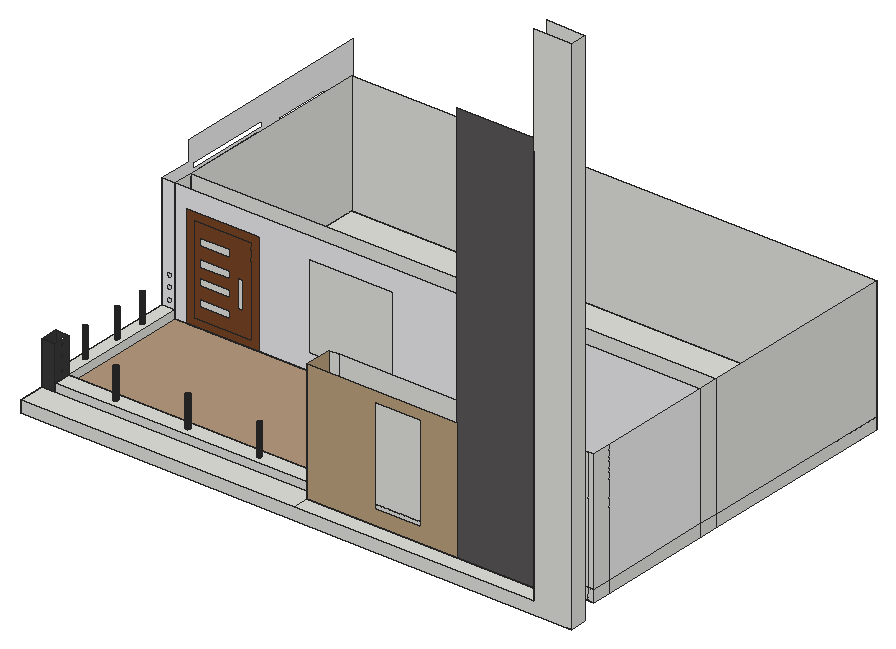
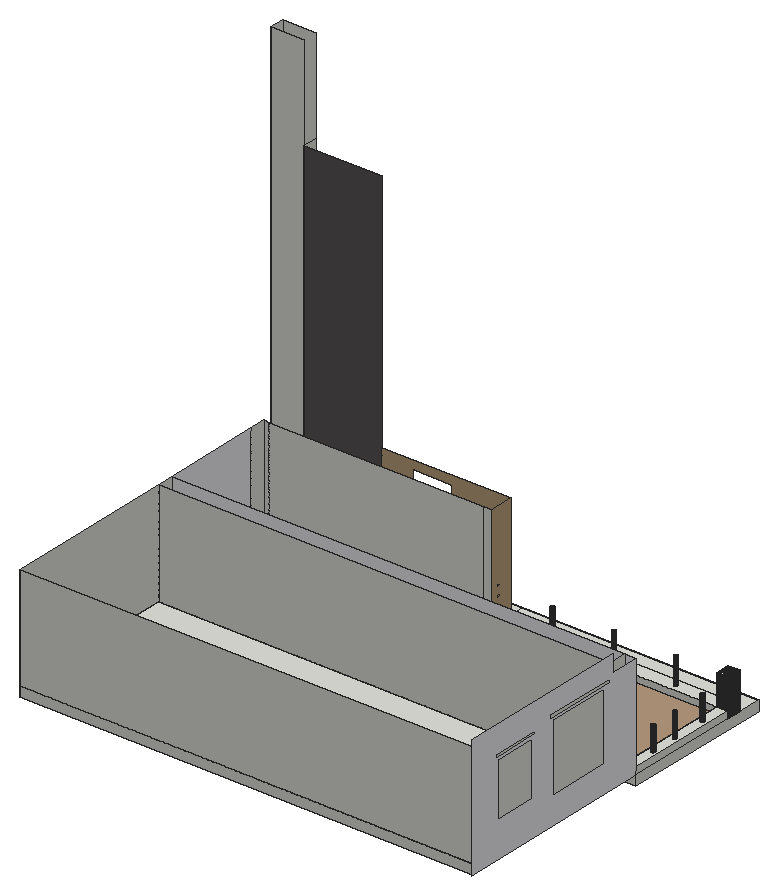
# SketchUp Ruby script. Lengths in inches.
U = 1.inch
M = Sketchup.active_model
def pt(a) = Geom::Point3d.new(a.map { |v| v * U })
def face(e, loops, mat)
  f = e.add_face(loops[0].map { |a| pt(a) })
  loops[1..].each { |l| e.add_face(l.map { |a| pt(a) }).erase! }
  f.material = f.back_material = mat if mat
  f
end
# faces: each face lists its corners as indices into pts; further lists are holes
def faces(e, pts, list, mat = nil) = list.each { |f| face(e, (f[0].is_a?(Array) ? f : [f]).map { |l| l.map { |i| pts[i] } }, mat) }
# xy, xz, yz: faces in a plane at the given z, y or x. An outline is a flat list of corners, or four numbers for a rectangle; further outlines are holes
def ring(l) = l.size == 4 ? [[l[0], l[1]], [l[2], l[1]], [l[2], l[3]], [l[0], l[3]]] : l.each_slice(2).to_a
def flat(e, list, mat, &to3) = list.each { |f| face(e, (f[0].is_a?(Array) ? f : [f]).map { |l| ring(l).map { |u, v| to3.(u, v) } }, mat) }
def xy(e, z, list, mat = nil) = flat(e, list, mat) { |x, y| [x, y, z] }
def xz(e, y, list, mat = nil) = flat(e, list, mat) { |x, z| [x, y, z] }
def yz(e, x, list, mat = nil) = flat(e, list, mat) { |y, z| [x, y, z] }
def lines(e, pts, list) = list.each { |a, b| e.add_line(pt(pts[a]), pt(pts[b])) }
# prism: a flat outline (further loops are holes) pulled along v
def prism(e, loops, v, mat = nil)
  f = face(e, loops, mat); d = Geom::Vector3d.new(v.map { |x| x * U })
  f.pushpull(f.normal.samedirection?(d) ? d.length : -d.length)
end
def box(e, o, s, mat = nil) = prism(e, [[o, [o[0] + s[0], o[1], o[2]], [o[0] + s[0], o[1] + s[1], o[2]], [o[0], o[1] + s[1], o[2]]]], [0, 0, s[2]], mat)
def at(x, y, z, deg = 0) = Geom::Transformation.translation(pt([x, y, z])) * Geom::Transformation.rotation(ORIGIN, Z_AXIS, deg.degrees)
def axes(o, x, y, z) = Geom::Transformation.new([*x, 0, *y, 0, *z, 0, *pt(o).to_a, 1])
def part(name) = M.definitions.add(name)
# library, detail: a bought-in or finely detailed component or shape, given as its bounding box
def library(name, o, s) = part(name).tap { |d| box(d.entities, o, s) }
def detail(e, o, s) = box(e.add_group.entities, o, s)
def put(e, d, t, mat = nil) = e.add_instance(d, t).tap { |i| i.material = mat if mat }
def group(e, t, mat = nil) = e.add_group.tap { |g| g.transformation = t; g.material = mat if mat }.entities
root = M.entities
M.materials.add("[0035_Tan]").color = [188, 161, 125]
M.materials.add("[Blinds Vertical Pattern]").color = [237, 237, 239]
M.materials.add("[Blinds Vertical Pattern]1").color = [212, 212, 214]
M.materials.add("[Brick Tumbled]").color = [89, 87, 87]
M.materials.add("[Carpet Pattern Leaf Squares Tan]").color = [181, 154, 125]
M.materials.add("[Color M07]").color = [58, 58, 58]
M.materials.add("[Wood Veneer 01]").color = [120, 70, 37]
xy(root,501.625,[[320.99,378.34,537.68,393.34],[537.68,378.34,572.32,393.34],[85.98,538.2,560.26,556.28],[85.98,556.28,560.26,737.09]])
xy(root,501.625,[[73.92,378.34,73.92,538.2,560.26,538.2,560.26,418.04,320.99,418.04,320.99,378.34]],"[Blinds Vertical Pattern]1")
xy(root,512.25,[[73.92,378.34,320.99,402.63],[320.99,378.34,537.68,393.34],[73.92,402.63,85.98,418.04],[85.98,402.63,320.99,418.04],[73.92,418.04,85.98,538.2],
  [85.98,538.2,560.26,556.28],[85.98,556.28,560.26,737.09]])
xy(root,512.25,[[85.98,418.04,560.26,538.2]],"[Carpet Pattern Leaf Squares Tan]")
xy(root,519.4375,[[[85.98,402.63,320.99,418.04],[134.48,408.67,134.01,408.73,133.58,408.91,133.2,409.2,132.91,409.58,132.73,410.01,132.67,410.48,132.73,410.95,132.91,411.39,133.2,411.76,133.58,412.05,134.01,412.23,134.48,412.3,134.95,412.23,135.39,412.05,135.76,411.76,136.05,411.39,136.23,410.95,136.29,410.48,136.23,410.01,136.05,409.58,135.76,409.2,135.39,408.91,134.95,408.73],[264.29,408.67,263.82,408.73,263.39,408.91,263.01,409.2,262.72,409.58,262.54,410.01,262.48,410.48,262.54,410.95,262.72,411.39,263.01,411.76,263.39,412.05,263.82,412.23,264.29,412.3,264.76,412.23,265.2,412.05,265.58,411.76,265.86,411.39,266.04,410.95,266.11,410.48,266.04,410.01,265.86,409.58,265.58,409.2,265.2,408.91,264.76,408.73],[199.54,408.67,199.07,408.73,198.64,408.91,198.26,409.2,197.97,409.58,197.79,410.01,197.73,410.48,197.79,410.95,197.97,411.39,198.26,411.76,198.64,412.05,199.07,412.23,199.54,412.3,200.01,412.23,200.45,412.05,200.83,411.76,201.11,411.39,201.29,410.95,201.36,410.48,201.29,410.01,201.11,409.58,200.83,409.2,200.45,408.91,200.01,408.73]],[134.48,408.67,134.01,408.73,133.58,408.91,133.2,409.2,132.91,409.58,132.73,410.01,132.67,410.48,132.73,410.95,132.91,411.39,133.2,411.76,133.58,412.05,134.01,412.23,134.48,412.3,134.95,412.23,135.39,412.05,135.76,411.76,136.05,411.39,136.23,410.95,136.29,410.48,136.23,410.01,136.05,409.58,135.76,409.2,135.39,408.91,134.95,408.73],[199.54,408.67,199.07,408.73,198.64,408.91,198.26,409.2,197.97,409.58,197.79,410.01,197.73,410.48,197.79,410.95,197.97,411.39,198.26,411.76,198.64,412.05,199.07,412.23,199.54,412.3,200.01,412.23,200.45,412.05,200.83,411.76,201.11,411.39,201.29,410.95,201.36,410.48,201.29,410.01,201.11,409.58,200.83,409.2,200.45,408.91,200.01,408.73],[264.29,408.67,263.82,408.73,263.39,408.91,263.01,409.2,262.72,409.58,262.54,410.01,262.48,410.48,262.54,410.95,262.72,411.39,263.01,411.76,263.39,412.05,263.82,412.23,264.29,412.3,264.76,412.23,265.2,412.05,265.58,411.76,265.86,411.39,266.04,410.95,266.11,410.48,266.04,410.01,265.86,409.58,265.58,409.2,265.2,408.91,264.76,408.73],[[73.92,418.04,85.98,538.2],[79.76,442.375,79.29,442.4375,78.85,442.62,78.48,442.91,78.1875,443.28,78.01,443.72,77.95,444.1875,78.01,444.66,78.1875,445.09,78.48,445.47,78.85,445.76,79.29,445.9375,79.76,446,80.23,445.9375,80.66,445.76,81.04,445.47,81.33,445.09,81.51,444.66,81.57,444.1875,81.51,443.72,81.33,443.28,81.04,442.91,80.66,442.62,80.23,442.4375],[79.76,506.9375,79.29,507,78.85,507.18,78.48,507.47,78.1875,507.84,78.01,508.28,77.95,508.75,78.01,509.22,78.1875,509.66,78.48,510.03,78.85,510.32,79.29,510.5,79.76,510.5625,80.23,510.5,80.66,510.32,81.04,510.03,81.33,509.66,81.51,509.22,81.57,508.75,81.51,508.28,81.33,507.84,81.04,507.47,80.66,507.18,80.23,507],[79.76,478.5,79.29,478.5625,78.85,478.74,78.48,479.03,78.1875,479.41,78.01,479.84,77.95,480.3125,78.01,480.78,78.1875,481.22,78.48,481.6,78.85,481.88,79.29,482.0625,79.76,482.125,80.23,482.0625,80.66,481.88,81.04,481.6,81.33,481.22,81.51,480.78,81.57,480.3125,81.51,479.84,81.33,479.41,81.04,479.03,80.66,478.74,80.23,478.5625]],
  [79.76,442.375,79.29,442.4375,78.85,442.62,78.48,442.91,78.1875,443.28,78.01,443.72,77.95,444.1875,78.01,444.66,78.1875,445.09,78.48,445.47,78.85,445.76,79.29,445.9375,79.76,446,80.23,445.9375,80.66,445.76,81.04,445.47,81.33,445.09,81.51,444.66,81.57,444.1875,81.51,443.72,81.33,443.28,81.04,442.91,80.66,442.62,80.23,442.4375],[79.76,478.5,79.29,478.5625,78.85,478.74,78.48,479.03,78.1875,479.41,78.01,479.84,77.95,480.3125,78.01,480.78,78.1875,481.22,78.48,481.6,78.85,481.88,79.29,482.0625,79.76,482.125,80.23,482.0625,80.66,481.88,81.04,481.6,81.33,481.22,81.51,480.78,81.57,480.3125,81.51,479.84,81.33,479.41,81.04,479.03,80.66,478.74,80.23,478.5625],[79.76,506.9375,79.29,507,78.85,507.18,78.48,507.47,78.1875,507.84,78.01,508.28,77.95,508.75,78.01,509.22,78.1875,509.66,78.48,510.03,78.85,510.32,79.29,510.5,79.76,510.5625,80.23,510.5,80.66,510.32,81.04,510.03,81.33,509.66,81.51,509.22,81.57,508.75,81.51,508.28,81.33,507.84,81.04,507.47,80.66,507.18,80.23,507]])
xz(root,378.34,[[73.92,501.625,572.32,501.625,572.32,975.8,537.68,975.8,537.68,512.25,73.92,512.25]])
xz(root,393.34,[[320.99,501.625,320.99,512.25,537.68,512.25,537.68,975.8,572.32,975.8,572.32,501.625]])
xz(root,393.34,[[[320.99,512.25,456.39,621.625],[382.62,525.6875,423.93,612.6875]]],"[0035_Tan]")
xz(root,393.34,[[456.39,512.25,537.68,876.375]],"[Brick Tumbled]")
xz(root,402.63,[[85.98,512.25,320.99,519.4375]])
xz(root,402.63,[[73.92,512.25,85.98,551.25]],"[Color M07]")
xz(root,418.04,[[320.99,501.625,329.72,512.25],[329.72,501.625,554.62,512.25],[554.62,501.625,560.26,512.25],[73.92,512.25,85.98,519.4375],[85.98,512.25,320.99,519.4375],
  [320.99,512.25,329.72,621.625],[329.72,512.25,554.62,621.625],[554.62,512.25,560.26,621.625]])
xz(root,418.04,[[[73.92,519.4375,85.98,551.25],[80.8,522.8,81.41,522.89,81.99,523.12,82.48,523.5,82.85,523.99,83.09,524.5625,83.17,525.18,83.09,525.79,82.85,526.37,82.48,526.86,81.99,527.24,81.41,527.47,80.8,527.55,80.18,527.47,79.61,527.24,79.12,526.86,78.74,526.37,78.5,525.79,78.42,525.18,78.5,524.5625,78.74,523.99,79.12,523.5,79.61,523.12,80.18,522.89],[80.8,533.37,81.41,533.45,81.99,533.68,82.48,534.0625,82.85,534.55,83.09,535.125,83.17,535.74,83.09,536.36,82.85,536.93,82.48,537.42,81.99,537.8,81.41,538.04,80.8,538.12,80.18,538.04,79.61,537.8,79.12,537.42,78.74,536.93,78.5,536.36,78.42,535.74,78.5,535.125,78.74,534.55,79.12,534.0625,79.61,533.68,80.18,533.45],[80.8,543.3,81.41,543.39,81.99,543.62,82.48,544,82.85,544.49,83.09,545.0625,83.17,545.68,83.09,546.29,82.85,546.87,82.48,547.36,81.99,547.74,81.41,547.97,80.8,548.05,80.18,547.97,79.61,547.74,79.12,547.36,78.74,546.87,78.5,546.29,78.42,545.68,78.5,545.0625,78.74,544.49,79.12,544,79.61,543.62,80.18,543.39]]],"[Color M07]")
xz(root,538.2,[[73.92,501.625,85.98,512.25],[85.98,501.625,560.26,512.25],[73.92,512.25,85.98,519.4375]])
xz(root,538.2,[[[85.98,512.25,96.7,512.25,96.7,604.625,161.2,604.625,161.2,512.25,560.26,512.25,560.26,621.625,85.98,621.625],[206.59,526.85,282.28,602.54]],[[73.92,519.4375,85.98,621.625],[80.8,522.8,80.18,522.89,79.61,523.12,79.12,523.5,78.74,523.99,78.5,524.5625,78.42,525.18,78.5,525.79,78.74,526.37,79.12,526.86,79.61,527.24,80.18,527.47,80.8,527.55,81.41,527.47,81.99,527.24,82.48,526.86,82.85,526.37,83.09,525.79,83.17,525.18,83.09,524.5625,82.85,523.99,82.48,523.5,81.99,523.12,81.41,522.89],[80.8,543.3,80.18,543.39,79.61,543.62,79.12,544,78.74,544.49,78.5,545.0625,78.42,545.68,78.5,546.29,78.74,546.87,79.12,547.36,79.61,547.74,80.18,547.97,80.8,548.05,81.41,547.97,81.99,547.74,82.48,547.36,82.85,546.87,83.09,546.29,83.17,545.68,83.09,545.0625,82.85,544.49,82.48,544,81.99,543.62,81.41,543.39],[80.8,533.37,80.18,533.45,79.61,533.68,79.12,534.0625,78.74,534.55,78.5,535.125,78.42,535.74,78.5,536.36,78.74,536.93,79.12,537.42,79.61,537.8,80.18,538.04,80.8,538.12,81.41,538.04,81.99,537.8,82.48,537.42,82.85,536.93,83.09,536.36,83.17,535.74,83.09,535.125,82.85,534.55,82.48,534.0625,81.99,533.68,81.41,533.45]]],"[Blinds Vertical Pattern]")
xz(root,538.2,[[[96.7,512.25,161.2,604.625],[103.6,519.15,154.3,597.73]],[[103.6,519.15,154.3,597.73],[108.19,579.01,135.69,585.69],[108.19,529.57,135.69,536.26],[108.19,561.38,135.69,568.07],[108.19,546.38,135.69,553.07],[142.77,540.02,146.77,565.12]]],"[Wood Veneer 01]")
xz(root,556.28,[[85.98,501.625,560.26,512.25],[85.98,512.25,560.26,621.625]])
xz(root,737.09,[[85.98,501.625,560.26,512.25],[85.98,512.25,560.26,621.625]])
yz(root,73.92,[[378.34,501.625,538.2,512.25],[418.04,512.25,538.2,519.4375]])
yz(root,73.92,[[[538.2,512.25,538.2,621.625,568.32,621.625,568.32,639.5625,753.91,639.5625,753.91,512.25],[580.21,541.0625,647.71,611.8125],[674.43,550.0625,719.61,606.375],[573.4375,613.9375,651,618.1875],[670.75,608.8,722.6875,612.23]]],"[Blinds Vertical Pattern]")
yz(root,73.92,[[402.63,512.25,418.04,551.25]],"[Color M07]")
yz(root,85.98,[[538.2,501.625,556.28,512.25],[556.28,501.625,737.09,512.25],[402.63,512.25,418.04,519.4375],[418.04,512.25,538.2,519.4375],[538.2,512.25,556.28,621.625],
  [556.28,512.25,737.09,621.625]])
yz(root,85.98,[[[402.63,519.4375,418.04,551.25],[410.2,545.51,409.75,545.57,409.33,545.74,408.97,546.02,408.6875,546.38,408.51,546.8,408.45,547.26,408.51,547.71,408.6875,548.13,408.97,548.49,409.33,548.77,409.75,548.95,410.2,549.01,410.66,548.95,411.08,548.77,411.44,548.49,411.72,548.13,411.89,547.71,411.95,547.26,411.89,546.8,411.72,546.38,411.44,546.02,411.08,545.74,410.66,545.57],[410.2,524.19,409.75,524.25,409.33,524.43,408.97,524.71,408.6875,525.07,408.51,525.49,408.45,525.94,408.51,526.4,408.6875,526.82,408.97,527.18,409.33,527.46,409.75,527.64,410.2,527.69,410.66,527.64,411.08,527.46,411.44,527.18,411.72,526.82,411.89,526.4,411.95,525.94,411.89,525.49,411.72,525.07,411.44,524.71,411.08,524.43,410.66,524.25],[410.2,535.38,409.75,535.44,409.33,535.62,408.97,535.89,408.6875,536.26,408.51,536.68,408.45,537.13,408.51,537.59,408.6875,538.01,408.97,538.37,409.33,538.65,409.75,538.82,410.2,538.88,410.66,538.82,411.08,538.65,411.44,538.37,411.72,538.01,411.89,537.59,411.95,537.13,411.89,536.68,411.72,536.26,411.44,535.89,411.08,535.62,410.66,535.44]]],"[Color M07]")
yz(root,320.99,[[393.34,501.625,418.04,512.25],[402.63,512.25,418.04,519.4375]])
yz(root,320.99,[[[393.34,512.25,393.34,621.625,418.04,621.625,418.04,519.4375,402.63,519.4375,402.63,512.25],[410.2,545.51,410.66,545.57,411.08,545.74,411.44,546.02,411.72,546.38,411.89,546.8,411.95,547.26,411.89,547.71,411.72,548.13,411.44,548.49,411.08,548.77,410.66,548.95,410.2,549.01,409.75,548.95,409.33,548.77,408.97,548.49,408.6875,548.13,408.51,547.71,408.45,547.26,408.51,546.8,408.6875,546.38,408.97,546.02,409.33,545.74,409.75,545.57],[410.2,535.38,410.66,535.44,411.08,535.62,411.44,535.89,411.72,536.26,411.89,536.68,411.95,537.13,411.89,537.59,411.72,538.01,411.44,538.37,411.08,538.65,410.66,538.82,410.2,538.88,409.75,538.82,409.33,538.65,408.97,538.37,408.6875,538.01,408.51,537.59,408.45,537.13,408.51,536.68,408.6875,536.26,408.97,535.89,409.33,535.62,409.75,535.44],[410.2,524.19,410.66,524.25,411.08,524.43,411.44,524.71,411.72,525.07,411.89,525.49,411.95,525.94,411.89,526.4,411.72,526.82,411.44,527.18,411.08,527.46,410.66,527.64,410.2,527.69,409.75,527.64,409.33,527.46,408.97,527.18,408.6875,526.82,408.51,526.4,408.45,525.94,408.51,525.49,408.6875,525.07,408.97,524.71,409.33,524.43,409.75,524.25]]],"[0035_Tan]")
yz(root,537.68,[[378.34,512.25,393.34,876.375]])
yz(root,560.26,[[418.04,501.625,434.85,512.25],[434.85,501.625,538.2,512.25],[538.2,501.625,556.28,512.25],[556.28,501.625,737.09,512.25],[418.04,512.25,434.85,621.625],
  [538.2,512.25,556.28,621.625],[556.28,512.25,737.09,621.625]])
yz(root,560.26,[[434.85,512.25,538.2,621.625]],"[Blinds Vertical Pattern]")
yz(root,572.32,[[378.34,501.625,393.34,975.8]])
p = [[133.58,408.91,519.4375],[134.01,408.73,519.4375],[134.01,408.73,546.625],[133.58,408.91,546.625],[134.48,408.67,519.4375],[134.48,408.67,546.625],
  [134.95,408.73,519.4375],[134.95,408.73,546.625],[135.39,408.91,519.4375],[135.39,408.91,546.625],[198.64,408.91,519.4375],[199.07,408.73,519.4375],
  [199.07,408.73,547.26],[198.64,408.91,547.26],[199.54,408.67,519.4375],[199.54,408.67,547.26],[200.01,408.73,519.4375],[200.01,408.73,547.26],
  [200.45,408.91,519.4375],[200.45,408.91,547.26],[263.39,408.91,519.4375],[263.82,408.73,519.4375],[263.82,408.73,547.125],[263.39,408.91,547.125],
  [264.29,408.67,519.4375],[264.29,408.67,547.125],[264.76,408.73,519.4375],[264.76,408.73,547.125],[265.2,408.91,519.4375],[265.2,408.91,547.125],
  [133.2,409.2,519.4375],[133.2,409.2,546.625],[135.76,409.2,519.4375],[135.76,409.2,546.625],[198.26,409.2,519.4375],[198.26,409.2,547.26],
  [200.83,409.2,519.4375],[200.83,409.2,547.26],[263.01,409.2,519.4375],[263.01,409.2,547.125],[265.58,409.2,519.4375],[265.58,409.2,547.125],
  [132.91,409.58,519.4375],[132.91,409.58,546.625],[136.05,409.58,519.4375],[136.05,409.58,546.625],[197.97,409.58,519.4375],[197.97,409.58,547.26],
  [201.11,409.58,519.4375],[201.11,409.58,547.26],[262.72,409.58,519.4375],[262.72,409.58,547.125],[265.86,409.58,519.4375],[265.86,409.58,547.125],
  [132.73,410.01,519.4375],[132.73,410.01,546.625],[136.23,410.01,519.4375],[136.23,410.01,546.625],[197.79,410.01,519.4375],[197.79,410.01,547.26],
  [201.29,410.01,519.4375],[201.29,410.01,547.26],[262.54,410.01,519.4375],[262.54,410.01,547.125],[266.04,410.01,519.4375],[266.04,410.01,547.125],
  [132.67,410.48,519.4375],[132.67,410.48,546.625],[136.29,410.48,519.4375],[136.29,410.48,546.625],[197.73,410.48,519.4375],[197.73,410.48,547.26],
  [201.36,410.48,519.4375],[201.36,410.48,547.26],[262.48,410.48,519.4375],[262.48,410.48,547.125],[266.11,410.48,519.4375],[266.11,410.48,547.125],
  [132.73,410.95,519.4375],[132.73,410.95,546.625],[136.23,410.95,519.4375],[136.23,410.95,546.625],[197.79,410.95,519.4375],[197.79,410.95,547.26],
  [201.29,410.95,519.4375],[201.29,410.95,547.26],[262.54,410.95,519.4375],[262.54,410.95,547.125],[266.04,410.95,519.4375],[266.04,410.95,547.125],
  [132.91,411.39,519.4375],[132.91,411.39,546.625],[136.05,411.39,519.4375],[136.05,411.39,546.625],[197.97,411.39,519.4375],[197.97,411.39,547.26],
  [201.11,411.39,519.4375],[201.11,411.39,547.26],[262.72,411.39,519.4375],[262.72,411.39,547.125],[265.86,411.39,519.4375],[265.86,411.39,547.125],
  [133.2,411.76,519.4375],[133.2,411.76,546.625],[135.76,411.76,519.4375],[135.76,411.76,546.625],[198.26,411.76,519.4375],[198.26,411.76,547.26],
  [200.83,411.76,519.4375],[200.83,411.76,547.26],[263.01,411.76,519.4375],[263.01,411.76,547.125],[265.58,411.76,519.4375],[265.58,411.76,547.125],
  [133.58,412.05,519.4375],[133.58,412.05,546.625],[135.39,412.05,519.4375],[135.39,412.05,546.625],[198.64,412.05,519.4375],[198.51,411.95,547.26],
  [198.64,412.05,547.26],[200.45,412.05,519.4375],[200.45,412.05,547.26],[200.58,411.95,547.26],[263.39,412.05,519.4375],[263.39,412.05,547.125],
  [265.2,412.05,519.4375],[265.2,412.05,547.125],[134.01,412.23,519.4375],[134.01,412.23,546.625],[134.95,412.23,519.4375],[134.95,412.23,546.625],
  [199.07,412.23,519.4375],[199.07,412.23,547.26],[200.01,412.23,519.4375],[200.01,412.23,547.26],[263.82,412.23,519.4375],[263.82,412.23,547.125],
  [264.76,412.23,519.4375],[264.76,412.23,547.125],[134.48,412.3,519.4375],[134.48,412.3,546.625],[199.54,412.3,519.4375],[199.54,412.3,547.26],
  [264.29,412.3,519.4375],[264.29,412.3,547.125],[78.85,442.62,519.4375],[79.29,442.4375,519.4375],[79.29,442.4375,545.3125],[78.85,442.62,545.3125],
  [79.76,442.375,519.4375],[79.76,442.375,545.3125],[80.23,442.4375,519.4375],[80.23,442.4375,545.3125],[80.66,442.62,519.4375],[80.66,442.62,545.3125],
  [78.48,442.91,519.4375],[78.48,442.91,545.3125],[81.04,442.91,519.4375],[81.04,442.91,545.3125],[78.1875,443.28,519.4375],[78.1875,443.28,545.3125],
  [81.33,443.28,519.4375],[81.33,443.28,545.3125],[78.01,443.72,519.4375],[78.01,443.72,545.3125],[81.51,443.72,519.4375],[81.51,443.72,545.3125],
  [77.95,444.1875,519.4375],[77.95,444.1875,545.3125],[81.57,444.1875,519.4375],[81.57,444.1875,545.3125],[78.01,444.66,519.4375],[78.01,444.66,545.3125],
  [81.51,444.66,519.4375],[81.51,444.66,545.3125],[78.1875,445.09,519.4375],[78.1875,445.09,545.3125],[81.33,445.09,519.4375],[81.33,445.09,545.3125],
  [78.48,445.47,519.4375],[78.48,445.47,545.3125],[81.04,445.47,519.4375],[81.04,445.47,545.3125],[78.85,445.76,519.4375],[78.85,445.76,545.3125],
  [80.66,445.76,519.4375],[80.66,445.76,545.3125],[79.29,445.9375,519.4375],[79.29,445.9375,545.3125],[80.23,445.9375,519.4375],[80.23,445.9375,545.3125],
  [79.76,446,519.4375],[79.76,446,545.3125],[79.29,478.5625,519.4375],[79.76,478.5,519.4375],[79.76,478.5,544.75],[79.29,478.5625,544.75],
  [80.23,478.5625,519.4375],[80.23,478.5625,544.75],[78.85,478.74,519.4375],[78.85,478.74,544.75],[80.66,478.74,519.4375],[80.66,478.74,544.75],
  [78.48,479.03,519.4375],[78.48,479.03,544.75],[81.04,479.03,519.4375],[81.04,479.03,544.75],[78.1875,479.41,519.4375],[78.1875,479.41,544.75],
  [81.33,479.41,519.4375],[81.33,479.41,544.75],[78.01,479.84,519.4375],[78.01,479.84,544.75],[81.51,479.84,519.4375],[81.51,479.84,544.75],
  [77.95,480.3125,519.4375],[77.95,480.3125,544.75],[81.57,480.3125,519.4375],[81.57,480.3125,544.75],[78.01,480.78,519.4375],[78.01,480.78,544.75],
  [81.51,480.78,519.4375],[81.51,480.78,544.75],[78.1875,481.22,519.4375],[78.1875,481.22,544.75],[81.33,481.22,519.4375],[81.33,481.22,544.75],
  [78.48,481.6,519.4375],[78.48,481.6,544.75],[81.04,481.6,519.4375],[81.04,481.6,544.75],[78.85,481.88,519.4375],[78.85,481.88,544.75],
  [80.66,481.88,519.4375],[80.66,481.88,544.75],[79.29,482.0625,519.4375],[79.29,482.0625,544.75],[80.23,482.0625,519.4375],[80.23,482.0625,544.75],
  [79.76,482.125,519.4375],[79.76,482.125,544.75],[79.29,507,519.4375],[79.76,506.9375,519.4375],[79.76,506.9375,544.4375],[79.29,507,544.4375],
  [80.23,507,519.4375],[80.23,507,544.4375],[78.85,507.18,519.4375],[78.85,507.18,544.4375],[80.66,507.18,519.4375],[80.66,507.18,544.4375],
  [78.48,507.47,519.4375],[78.48,507.47,544.4375],[81.04,507.47,519.4375],[81.04,507.47,544.4375],[78.1875,507.84,519.4375],[78.1875,507.84,544.4375],
  [81.33,507.84,519.4375],[81.33,507.84,544.4375],[78.01,508.28,519.4375],[78.01,508.28,544.4375],[81.51,508.28,519.4375],[81.51,508.28,544.4375],
  [77.95,508.75,519.4375],[77.95,508.75,544.4375],[81.57,508.75,519.4375],[81.57,508.75,544.4375],[78.01,509.22,519.4375],[78.01,509.22,544.4375],
  [81.51,509.22,519.4375],[81.51,509.22,544.4375],[78.1875,509.66,519.4375],[78.1875,509.66,544.4375],[81.33,509.66,519.4375],[81.33,509.66,544.4375],
  [78.48,510.03,519.4375],[78.48,510.03,544.4375],[81.04,510.03,519.4375],[81.04,510.03,544.4375],[78.85,510.32,519.4375],[78.85,510.32,544.4375],
  [80.66,510.32,519.4375],[80.66,510.32,544.4375],[79.29,510.5,519.4375],[79.29,510.5,544.4375],[80.23,510.5,519.4375],[80.23,510.5,544.4375],
  [79.76,510.5625,519.4375],[79.76,510.5625,544.4375]]
faces(root,p,[[0,1,2,3],[1,4,5,2],[4,6,7,5],[6,8,9,7],[10,11,12,13],[11,14,15,12],[14,16,17,15],[16,18,19,17],
  [20,21,22,23],[21,24,25,22],[24,26,27,25],[26,28,29,27],[30,0,3,31],[8,32,33,9],[34,10,13,35],[18,36,37,19],
  [38,20,23,39],[28,40,41,29],[42,30,31,43],[32,44,45,33],[46,34,35,47],[36,48,49,37],[50,38,39,51],[40,52,53,41],
  [54,42,43,55],[44,56,57,45],[58,46,47,59],[48,60,61,49],[62,50,51,63],[52,64,65,53],[66,54,55,67],[56,68,69,57],
  [70,58,59,71],[60,72,73,61],[74,62,63,75],[64,76,77,65],[78,66,67,79],[68,80,81,69],[82,70,71,83],[72,84,85,73],
  [86,74,75,87],[76,88,89,77],[90,78,79,91],[80,92,93,81],[94,82,83,95],[84,96,97,85],[98,86,87,99],[88,100,101,89],
  [102,90,91,103],[92,104,105,93],[106,94,95,107],[96,108,109,97],[110,98,99,111],[100,112,113,101],[114,102,103,115],[104,116,117,105],
  [118,106,107,119,120],[108,121,122,123,109],[124,110,111,125],[112,126,127,113],[128,114,115,129],[116,130,131,117],[132,118,120,133],[121,134,135,122],
  [136,124,125,137],[126,138,139,127],[140,128,129,141],[130,140,141,131],[142,132,133,143],[134,142,143,135],[144,136,137,145],[138,144,145,139],
  [146,147,148,149],[147,150,151,148],[150,152,153,151],[152,154,155,153],[156,146,149,157],[154,158,159,155],[160,156,157,161],[158,162,163,159],
  [164,160,161,165],[162,166,167,163],[168,164,165,169],[166,170,171,167],[172,168,169,173],[170,174,175,171],[176,172,173,177],[174,178,179,175],
  [180,176,177,181],[178,182,183,179],[184,180,181,185],[182,186,187,183],[188,184,185,189],[186,190,191,187],[192,188,189,193],[190,192,193,191],
  [194,195,196,197],[195,198,199,196],[200,194,197,201],[198,202,203,199],[204,200,201,205],[202,206,207,203],[208,204,205,209],[206,210,211,207],
  [212,208,209,213],[210,214,215,211],[216,212,213,217],[214,218,219,215],[220,216,217,221],[218,222,223,219],[224,220,221,225],[222,226,227,223],
  [228,224,225,229],[226,230,231,227],[232,228,229,233],[230,234,235,231],[236,232,233,237],[234,238,239,235],[240,236,237,241],[238,240,241,239],
  [242,243,244,245],[243,246,247,244],[248,242,245,249],[246,250,251,247],[252,248,249,253],[250,254,255,251],[256,252,253,257],[254,258,259,255],
  [260,256,257,261],[258,262,263,259],[264,260,261,265],[262,266,267,263],[268,264,265,269],[266,270,271,267],[272,268,269,273],[270,274,275,271],
  [276,272,273,277],[274,278,279,275],[280,276,277,281],[278,282,283,279],[284,280,281,285],[282,286,287,283],[288,284,285,289],[286,288,289,287]],"[Color M07]")
